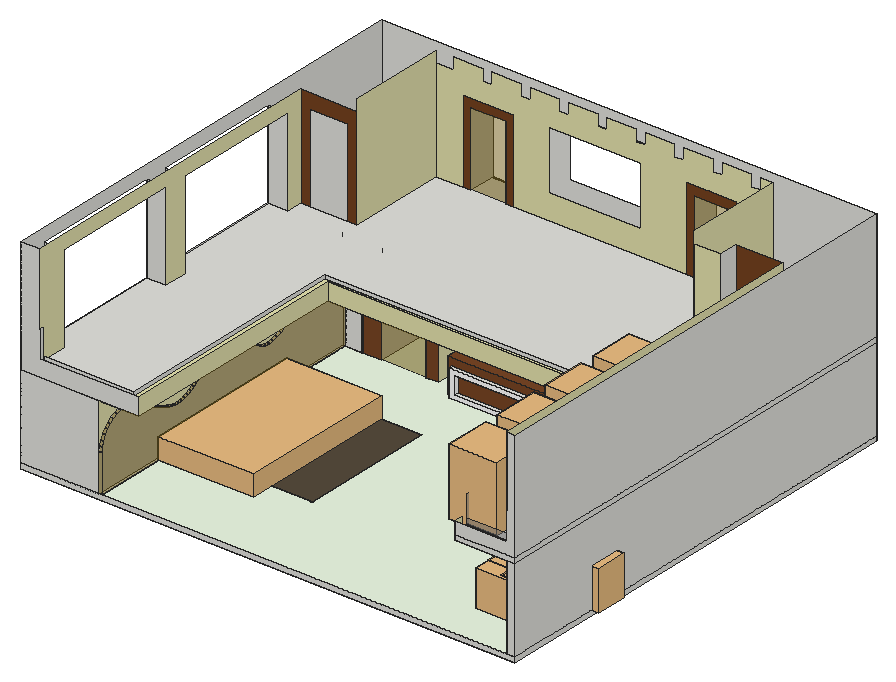
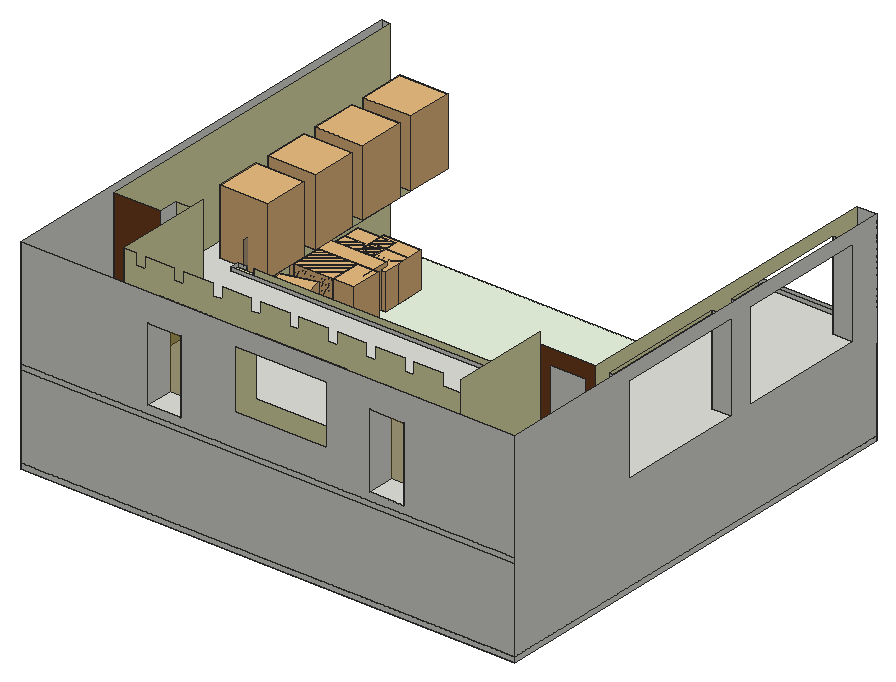
# SketchUp Ruby script. Lengths in inches.
U = 1.inch
M = Sketchup.active_model
def pt(a) = Geom::Point3d.new(a.map { |v| v * U })
def face(e, loops, mat)
  f = e.add_face(loops[0].map { |a| pt(a) })
  loops[1..].each { |l| e.add_face(l.map { |a| pt(a) }).erase! }
  f.material = f.back_material = mat if mat
  f
end
# faces: each face lists its corners as indices into pts; further lists are holes
def faces(e, pts, list, mat = nil) = list.each { |f| face(e, (f[0].is_a?(Array) ? f : [f]).map { |l| l.map { |i| pts[i] } }, mat) }
# xy, xz, yz: faces in a plane at the given z, y or x. An outline is a flat list of corners, or four numbers for a rectangle; further outlines are holes
def ring(l) = l.size == 4 ? [[l[0], l[1]], [l[2], l[1]], [l[2], l[3]], [l[0], l[3]]] : l.each_slice(2).to_a
def flat(e, list, mat, &to3) = list.each { |f| face(e, (f[0].is_a?(Array) ? f : [f]).map { |l| ring(l).map { |u, v| to3.(u, v) } }, mat) }
def xy(e, z, list, mat = nil) = flat(e, list, mat) { |x, y| [x, y, z] }
def xz(e, y, list, mat = nil) = flat(e, list, mat) { |x, z| [x, y, z] }
def yz(e, x, list, mat = nil) = flat(e, list, mat) { |y, z| [x, y, z] }
def lines(e, pts, list) = list.each { |a, b| e.add_line(pt(pts[a]), pt(pts[b])) }
# prism: a flat outline (further loops are holes) pulled along v
def prism(e, loops, v, mat = nil)
  f = face(e, loops, mat); d = Geom::Vector3d.new(v.map { |x| x * U })
  f.pushpull(f.normal.samedirection?(d) ? d.length : -d.length)
end
def box(e, o, s, mat = nil) = prism(e, [[o, [o[0] + s[0], o[1], o[2]], [o[0] + s[0], o[1] + s[1], o[2]], [o[0], o[1] + s[1], o[2]]]], [0, 0, s[2]], mat)
def at(x, y, z, deg = 0) = Geom::Transformation.translation(pt([x, y, z])) * Geom::Transformation.rotation(ORIGIN, Z_AXIS, deg.degrees)
def axes(o, x, y, z) = Geom::Transformation.new([*x, 0, *y, 0, *z, 0, *pt(o).to_a, 1])
def part(name) = M.definitions.add(name)
# library, detail: a bought-in or finely detailed component or shape, given as its bounding box
def library(name, o, s) = part(name).tap { |d| box(d.entities, o, s) }
def detail(e, o, s) = box(e.add_group.entities, o, s)
def put(e, d, t, mat = nil) = e.add_instance(d, t).tap { |i| i.material = mat if mat }
def group(e, t, mat = nil) = e.add_group.tap { |g| g.transformation = t; g.material = mat if mat }.entities
root = M.entities
M.materials.add("Generic").color = [229, 227, 174]
M.materials.add("[Carpet Diamond Olive]").color = [86, 76, 60]
M.materials.add("[Color M00]").color = [255, 255, 255]
M.materials.add("[Tile Limestone Large]").color = [236, 249, 228]
M.materials.add("[Translucent Glass Dark Green]").color = [135, 108, 20]
M.materials["[Translucent Glass Dark Green]"].alpha = 0.5
M.materials.add("[Translucent Glass Gray]").color = [128, 128, 128]
M.materials["[Translucent Glass Gray]"].alpha = 0.5
M.materials.add("[Wood Cherry Original]").color = [117, 66, 32]
M.materials.add("[Wood Veneer 01]").color = [120, 70, 37]
c1 = library("Group3\#1",[-238.15,54.18,0],[46.4,43.96,56.68])
c2 = library("Mesa PP75 Dining Table(beckup)",[0,0,0],[55.12,55.12,30.6875])
c3 = library("Plant+2 (1)",[-9.13,-9.52,0],[51.76,51.77,66.88])
c4 = library("Group\#6",[-0.47,-0.47,0],[175.35,198.73,37.5625])
c5 = library("1",[-11,-10.66,0],[22,21.32,33.52])
c6 = part("DDR842RVS01100X")
xy(c6.entities,0,[[-70.87,0,47.24,78.74]])
xy(c6.entities,0.39,[[-70.87,0,47.24,78.74]],"[Carpet Diamond Olive]")
xz(c6.entities,0,[[-70.87,0,47.24,0.39]])
xz(c6.entities,78.74,[[-70.87,0,47.24,0.39]])
yz(c6.entities,-70.87,[[0,0,78.74,0.39]])
yz(c6.entities,47.24,[[0,0,78.74,0.39]])
c7 = library("Flower_pot 07",[-1.21,-1.21,0],[8.32,8.32,4.71])
c8 = library("Plant",[-27.84,-31.84,-1.26],[68.28,70.82,154.38])
c9 = part("Group\#8")
xz(c9.entities,0,[[0,0,75.33,169.3125]],"[Translucent Glass Dark Green]")
xy(root,-12,[[0,0,1142.0625,1041.5]])
xy(root,0,[[0,0,182,0,182,701.375,227.9375,701.375,227.9375,701.68,228.24,701.68,228.24,701.375,273.88,701.375,273.88,831.5,375.13,831.5,375.13,701.375,404.03,701.375,404.03,830.0625,754.81,830.0625,754.81,849.8125,863.56,849.8125,863.56,701.375,931.8125,701.375,931.8125,828.25,1093.9375,828.25,1093.9375,701.375,1122.5625,701.375,1122.5625,0,1142.0625,0,1142.0625,1041.5,0,1041.5],[182,0,189.3125,701.375]])
xy(root,0,[[[189.3125,0,1122.5625,0,1122.5625,701.375,1093.9375,701.375,1093.9375,828.25,931.8125,828.25,931.8125,701.375,863.56,701.375,863.56,849.8125,754.81,849.8125,754.81,830.0625,404.03,830.0625,404.03,701.375,375.13,701.375,375.13,831.5,273.88,831.5,273.88,701.375,228.24,701.375,228.24,701.68,227.9375,701.68,227.9375,701.375,189.3125,701.375],[454.04,669.74,454.04,678.18,444.4,678.18,444.4,766.31,750.77,766.31,750.77,678.18,710.05,678.18,710.05,669.74]]],"[Tile Limestone Large]")
xy(root,11.125,[[467.72,669.74,710.05,678.18]])
xy(root,50.52,[[467.72,669.74,640.72,678.18]])
xy(root,61.64,[[454.04,669.74,640.72,678.18]])
xy(root,79.9375,[[444.4,678.18,750.77,766.31]],"[Wood Veneer 01]")
xy(root,133.0625,[[273.88,701.375,375.13,831.5]])
xy(root,141.1875,[[931.8125,701.375,1093.9375,828.25]])
xy(root,192,[[227.9375,701.375,228.24,701.68]])
xy(root,192,[[182,0,182,701.375,404.03,701.375,404.03,830.0625,754.81,830.0625,754.81,849.8125,863.56,849.8125,863.56,701.375,1122.5625,701.375,1122.5625,542.9375,274.125,542.9375,274.125,0],[1003,0,1122.5625,542.9375]],"Generic")
xy(root,222.75,[[45.5625,11.0625,253.5,11.0625,253.5,562.3125,1038.97,562.3125,1038.97,542.9375,1018.875,542.9375,1018.875,15.375,1122.5625,15.375,1122.5625,796.5,1014.875,796.5,1014.875,752.375,952.125,752.375,952.125,980.0625,847.11,980.0625,847.11,1041.5,771.78,1041.5,771.78,980.0625,335.28,980.0625,335.28,1041.5,255.99,1041.5,255.99,980.0625,175.5625,980.0625,175.5625,752.375,45.5625,752.375,45.5625,713.6,0,713.6,0,417.04,45.5625,417.04,45.5625,364.1,0,364.1,0,67.54,45.5625,67.54]])
xz(root,0,[[0,-12,1142.0625,0],[0,0,182,192],[1122.5625,0,1142.0625,192],[0,192,274.125,192,274.125,231.375,45.5625,231.375,45.5625,457.375,0,457.375],[1003,192,1142.0625,204],
  [1003,204,1142.0625,204,1142.0625,457.375,1122.5625,457.375,1122.5625,231.375,1003,231.375]])
xz(root,0,[[182,0,189.3125,86]],"[Translucent Glass Dark Green]")
xz(root,11.0625,[[45.5625,222.75,253.5,231.375]])
xz(root,15.375,[[1018.875,222.75,1122.5625,237.375]],"[Translucent Glass Gray]")
xz(root,67.54,[[0,222.75,45.5625,426.5625]])
xz(root,364.1,[[0,222.75,45.5625,426.5625]])
xz(root,417.04,[[0,222.75,45.5625,426.5625]])
xz(root,542.9375,[[1018.875,222.75,1038.97,231.375]])
xz(root,542.9375,[[274.125,192,1003,231.375]],"Generic")
xz(root,562.3125,[[253.5,222.75,1038.97,231.375]])
xz(root,669.74,[[454.04,0,710.05,0,710.05,11.125,467.72,11.125,467.72,50.52,640.72,50.52,640.72,61.64,454.04,61.64]],"[Color M00]")
xz(root,678.18,[[444.4,0,454.04,0,454.04,61.64,640.72,61.64,640.72,50.52,467.72,50.52,467.72,11.125,710.05,11.125,710.05,0,750.77,0,750.77,79.9375,444.4,79.9375]],"[Wood Veneer 01]")
xz(root,701.375,[[182,0,189.3125,132.8],[189.3125,0,227.9375,0,227.9375,192,182,192,182,132.8,189.3125,132.8]])
xz(root,701.375,[[863.56,0,911.78,192]],"Generic")
xz(root,701.375,[[911.78,0,931.8125,0,931.8125,141.1875,1093.9375,141.1875,1093.9375,0,1122.5625,0,1122.5625,192,911.78,192]],"[Wood Cherry Original]")
xz(root,701.375,[[228.24,0,273.88,0,273.88,133.0625,375.13,133.0625,375.13,0,404.03,0,404.03,192,228.24,192]],"[Wood Veneer 01]")
xz(root,701.68,[[227.9375,0,228.24,192]])
xz(root,713.6,[[0,222.75,45.5625,426.5625]])
xz(root,752.375,[[67.69,222.75,151.75,422.75]])
xz(root,752.375,[[952.125,222.75,1014.875,457.375]],"Generic")
xz(root,752.375,[[45.5625,222.75,67.69,222.75,67.69,422.75,151.75,422.75,151.75,222.75,175.5625,222.75,175.5625,457.375,45.5625,457.375]],"[Wood Cherry Original]")
xz(root,766.31,[[444.4,0,750.77,79.9375]])
xz(root,796.5,[[1014.875,222.75,1122.5625,457.375]],"[Wood Cherry Original]")
xz(root,828.25,[[931.8125,0,1093.9375,141.1875]])
xz(root,830.0625,[[404.03,39.25,754.81,45.5625],[404.03,78.375,754.81,84.6875],[404.03,117.5,754.81,123.8125],[404.03,156.625,754.81,162.9375],[404.03,162.9375,754.81,192]])
xz(root,830.0625,[[404.03,0,754.81,39.25],[404.03,45.5625,754.81,78.375],[404.03,84.6875,754.81,117.5],[404.03,123.8125,754.81,156.625]],"Generic")
xz(root,831.5,[[273.88,0,375.13,133.0625]])
xz(root,849.8125,[[754.81,0,863.56,39.29],[754.81,39.29,863.56,45.61],[754.81,78.4,863.56,84.72],[754.81,117.51,863.56,123.83],[754.81,156.625,863.56,162.9375]])
xz(root,849.8125,[[754.81,45.61,863.56,78.4],[754.81,84.72,863.56,117.51],[754.81,123.83,863.56,156.625],[754.81,162.9375,863.56,192]],"Generic")
xz(root,980.0625,[[[175.5625,222.75,236.76,222.75,236.76,413.27,354.51,413.27,354.51,222.75,750.57,222.75,750.57,413.27,868.32,413.27,868.32,222.75,952.125,222.75,952.125,483.5625,924.64,483.5625,924.64,457.375,902.01,457.375,902.01,483.5625,836.08,483.5625,836.08,457.375,813.45,457.375,813.45,483.5625,747.51,483.5625,747.51,457.375,724.89,457.375,724.89,483.5625,658.95,483.5625,658.95,457.375,636.33,457.375,636.33,483.5625,570.39,483.5625,570.39,457.375,547.76,457.375,547.76,483.5625,481.83,483.5625,481.83,457.375,459.2,457.375,459.2,483.5625,393.26,483.5625,393.26,457.375,370.64,457.375,370.64,483.5625,304.7,483.5625,304.7,457.375,282.08,457.375,282.08,483.5625,216.14,483.5625,216.14,457.375,175.5625,457.375],[434.63,279.55,646.76,416.17]]],"Generic")
xz(root,980.0625,[[236.76,222.75,255.99,222.75,255.99,394.04,335.28,394.04,335.28,222.75,354.51,222.75,354.51,413.27,236.76,413.27],[750.57,222.75,771.78,222.75,771.78,392.0625,847.11,392.0625,847.11,222.75,868.32,222.75,868.32,413.27,750.57,413.27]],"[Wood Cherry Original]")
xz(root,1041.5,[[0,-12,1142.0625,0],[0,0,1142.0625,192],[0,192,1142.0625,204],[[0,204,1142.0625,457.375],[434.63,279.55,646.76,416.17],[255.99,222.75,335.28,394.04],[771.78,222.75,847.11,392.0625]]])
yz(root,0,[[0,-12,1041.5,0],[[0,0,1041.5,457.375],[417.04,222.75,713.6,426.5625],[67.54,222.75,364.1,426.5625]]])
yz(root,45.5625,[[11.0625,222.75,67.54,222.75,67.54,426.5625,364.1,426.5625,364.1,222.75,417.04,222.75,417.04,426.5625,713.6,426.5625,713.6,222.75,752.375,222.75,752.375,457.375,0,457.375,0,293.625,11.0625,293.625]],"Generic")
yz(root,175.5625,[[752.375,222.75,980.0625,483.5625]],"Generic")
yz(root,182,[[0,0,0,86,1.01,97.52,4.02,108.68,8.92,119.14,15.58,128.59,23.79,136.73,33.28,143.32,43.79,148.14,54.97,151.0625,66.49,151.99,78,150.89,89.13,147.8,99.56,142.81,107.26,138.33,115.03,133.97,122.87,129.71,130.76,125.58,138.72,121.56,146.73,117.65,154.8,113.87,162.92,110.2,171.09,106.65,179.32,103.22,187.6,99.91,195.92,96.72,204.71,94.02,213.76,92.4,222.95,91.87,232.13,92.46,241.17,94.14,249.95,96.9,258.32,100.7,266.1875,105.47,273.42,111.16,279.91,117.68,285.57,124.92,290.32,132.8,298.0625,144.8,307.84,155.21,319.34,163.68,332.18,169.9375,345.93,173.78,360.16,175.07,374.38,173.78,388.13,169.9375,400.97,163.68,412.47,155.21,422.25,144.8,429.99,132.8,436.06,123.4,443.72,115.25,452.73,108.61,462.79,103.71,473.5625,100.7,484.71,99.6875,495.85,100.7,506.63,103.71,516.6875,108.61,525.69,115.25,533.36,123.4,539.42,132.8,548.4,146.72,559.74,158.78,573.07,168.61,587.96,175.86,603.91,180.3125,620.4,181.8125,636.89,180.3125,652.84,175.86,667.73,168.61,681.06,158.78,692.4,146.72,701.375,132.8,701.375,0]])
yz(root,182,[[0,86,1.01,97.52,4.02,108.68,8.92,119.14,15.58,128.59,23.79,136.73,33.28,143.32,43.79,148.14,54.97,151.0625,66.49,151.99,78,150.89,89.13,147.8,99.56,142.81,107.26,138.33,115.03,133.97,122.87,129.71,130.76,125.58,138.72,121.56,146.73,117.65,154.8,113.87,162.92,110.2,171.09,106.65,179.32,103.22,187.6,99.91,195.92,96.72,204.71,94.02,213.76,92.4,222.95,91.87,232.13,92.46,241.17,94.14,249.95,96.9,258.32,100.7,266.1875,105.47,273.42,111.16,279.91,117.68,285.57,124.92,290.32,132.8,298.0625,144.8,307.84,155.21,319.34,163.68,332.18,169.9375,345.93,173.78,360.16,175.07,374.38,173.78,388.13,169.9375,400.97,163.68,412.47,155.21,422.25,144.8,429.99,132.8,436.06,123.4,443.72,115.25,452.73,108.61,462.79,103.71,473.5625,100.7,484.71,99.6875,495.85,100.7,506.63,103.71,516.6875,108.61,525.69,115.25,533.36,123.4,539.42,132.8,548.4,146.72,559.74,158.78,573.07,168.61,587.96,175.86,603.91,180.3125,620.4,181.8125,636.89,180.3125,652.84,175.86,667.73,168.61,681.06,158.78,692.4,146.72,701.375,132.8,701.375,192,0,192]],"Generic")
yz(root,189.3125,[[0,0,701.375,0,701.375,132.8,692.4,146.72,681.06,158.78,667.73,168.61,652.84,175.86,636.89,180.3125,620.4,181.8125,603.91,180.3125,587.96,175.86,573.07,168.61,559.74,158.78,548.4,146.72,539.42,132.8,533.36,123.4,525.69,115.25,516.6875,108.61,506.63,103.71,495.85,100.7,484.71,99.6875,473.5625,100.7,462.79,103.71,452.73,108.61,443.72,115.25,436.06,123.4,429.99,132.8,422.25,144.8,412.47,155.21,400.97,163.68,388.13,169.9375,374.38,173.78,360.16,175.07,345.93,173.78,332.18,169.9375,319.34,163.68,307.84,155.21,298.0625,144.8,290.32,132.8,285.57,124.92,279.91,117.68,273.42,111.16,266.1875,105.47,258.32,100.7,249.95,96.9,241.17,94.14,232.13,92.46,222.95,91.87,213.76,92.4,204.71,94.02,195.92,96.72,187.6,99.91,179.32,103.22,171.09,106.65,162.92,110.2,154.8,113.87,146.73,117.65,138.72,121.56,130.76,125.58,122.87,129.71,115.03,133.97,107.26,138.33,99.56,142.81,89.13,147.8,78,150.89,66.49,151.99,54.97,151.0625,43.79,148.14,33.28,143.32,23.79,136.73,15.58,128.59,8.92,119.14,4.02,108.68,1.01,97.52,0,86]],"[Translucent Glass Dark Green]")
yz(root,227.9375,[[701.375,0,701.68,192]])
yz(root,228.24,[[701.375,0,701.68,192]])
yz(root,253.5,[[11.0625,222.75,562.3125,231.375]])
yz(root,255.99,[[980.0625,222.75,1041.5,394.04]])
yz(root,273.88,[[701.375,0,831.5,133.0625]])
yz(root,274.125,[[0,192,542.9375,231.375]],"Generic")
yz(root,335.28,[[980.0625,222.75,1041.5,394.04]])
yz(root,375.13,[[701.375,0,831.5,133.0625]])
yz(root,404.03,[[701.375,0,830.0625,192]],"Generic")
yz(root,444.4,[[678.18,0,766.31,79.9375]],"[Wood Veneer 01]")
yz(root,454.04,[[669.74,0,678.18,61.64]],"[Color M00]")
yz(root,467.72,[[669.74,11.125,678.18,50.52]],"[Color M00]")
yz(root,640.72,[[669.74,50.52,678.18,61.64]])
yz(root,710.05,[[669.74,0,678.18,11.125]])
yz(root,750.77,[[678.18,0,766.31,79.9375]],"[Wood Veneer 01]")
yz(root,754.81,[[830.0625,0,849.8125,123.8125],[830.0625,123.8125,849.8125,156.625],[830.0625,156.625,849.8125,162.9375],[830.0625,162.9375,849.8125,192]])
yz(root,771.78,[[980.0625,222.75,1041.5,392.0625]])
yz(root,847.11,[[980.0625,222.75,1041.5,392.0625]])
yz(root,863.56,[[701.375,0,849.8125,192]],"Generic")
yz(root,931.8125,[[701.375,0,828.25,141.1875]])
yz(root,952.125,[[752.375,222.75,980.0625,483.5625]],"Generic")
yz(root,1003,[[0,192,542.9375,231.375]],"Generic")
yz(root,1014.875,[[752.375,222.75,796.5,457.375]])
yz(root,1018.875,[[15.375,222.75,542.9375,222.75,542.9375,231.375,549.9375,231.375,549.9375,287.4375,15.375,287.4375]],"[Translucent Glass Gray]")
yz(root,1038.97,[[542.9375,222.75,562.3125,231.375]])
yz(root,1093.9375,[[701.375,0,828.25,141.1875]])
yz(root,1122.5625,[[0,0,701.375,192],[15.375,222.75,15.375,293.625,0,293.625,0,457.375,796.5,457.375,796.5,222.75]],"Generic")
yz(root,1142.0625,[[0,-12,1041.5,0],[0,0,1041.5,192],[0,192,1041.5,204],[0,204,1041.5,457.375]])
p = [[182,1.01,97.52],[182,0,86],[189.3125,0,86],[189.3125,1.01,97.52],[182,222.95,91.87],[182,213.76,92.4],
  [189.3125,213.76,92.4],[189.3125,222.95,91.87],[182,232.13,92.46],[189.3125,232.13,92.46],[182,204.71,94.02],[189.3125,204.71,94.02],
  [182,241.17,94.14],[189.3125,241.17,94.14],[182,195.92,96.72],[189.3125,195.92,96.72],[182,249.95,96.9],[189.3125,249.95,96.9],
  [182,187.6,99.91],[189.3125,187.6,99.91],[182,258.32,100.7],[189.3125,258.32,100.7],[182,4.02,108.68],[189.3125,4.02,108.68],
  [182,484.71,99.6875],[182,473.5625,100.7],[189.3125,473.5625,100.7],[189.3125,484.71,99.6875],[182,495.85,100.7],[189.3125,495.85,100.7],
  [182,179.32,103.22],[189.3125,179.32,103.22],[182,266.1875,105.47],[189.3125,266.1875,105.47],[182,462.79,103.71],[189.3125,462.79,103.71],
  [182,506.63,103.71],[189.3125,506.63,103.71],[182,171.09,106.65],[189.3125,171.09,106.65],[182,452.73,108.61],[189.3125,452.73,108.61],
  [182,516.6875,108.61],[189.3125,516.6875,108.61],[182,273.42,111.16],[189.3125,273.42,111.16],[182,162.92,110.2],[189.3125,162.92,110.2],
  [182,443.72,115.25],[189.3125,443.72,115.25],[182,525.69,115.25],[189.3125,525.69,115.25],[182,8.92,119.14],[189.3125,8.92,119.14],
  [182,154.8,113.87],[189.3125,154.8,113.87],[182,279.91,117.68],[189.3125,279.91,117.68],[182,146.73,117.65],[189.3125,146.73,117.65],
  [182,436.06,123.4],[189.3125,436.06,123.4],[182,533.36,123.4],[189.3125,533.36,123.4],[182,138.72,121.56],[189.3125,138.72,121.56],
  [182,285.57,124.92],[189.3125,285.57,124.92],[182,15.58,128.59],[189.3125,15.58,128.59],[182,130.76,125.58],[189.3125,130.76,125.58],
  [182,429.99,132.8],[189.3125,429.99,132.8],[182,539.42,132.8],[189.3125,539.42,132.8],[182,290.32,132.8],[189.3125,290.32,132.8],
  [182,122.87,129.71],[189.3125,122.87,129.71],[182,23.79,136.73],[189.3125,23.79,136.73],[182,115.03,133.97],[189.3125,115.03,133.97],
  [182,298.0625,144.8],[189.3125,298.0625,144.8],[182,422.25,144.8],[189.3125,422.25,144.8],[182,548.4,146.72],[189.3125,548.4,146.72],
  [182,701.375,132.8],[182,692.4,146.72],[189.3125,692.4,146.72],[189.3125,701.375,132.8],[182,107.26,138.33],[189.3125,107.26,138.33],
  [182,33.28,143.32],[189.3125,33.28,143.32],[182,99.56,142.81],[189.3125,99.56,142.81],[182,89.13,147.8],[189.3125,89.13,147.8],
  [182,43.79,148.14],[189.3125,43.79,148.14],[182,307.84,155.21],[189.3125,307.84,155.21],[182,412.47,155.21],[189.3125,412.47,155.21],
  [182,559.74,158.78],[189.3125,559.74,158.78],[182,681.06,158.78],[189.3125,681.06,158.78],[182,78,150.89],[189.3125,78,150.89],
  [182,54.97,151.0625],[189.3125,54.97,151.0625],[182,66.49,151.99],[189.3125,66.49,151.99],[182,319.34,163.68],[189.3125,319.34,163.68],
  [182,400.97,163.68],[189.3125,400.97,163.68],[182,573.07,168.61],[189.3125,573.07,168.61],[182,667.73,168.61],[189.3125,667.73,168.61],
  [182,332.18,169.9375],[189.3125,332.18,169.9375],[182,388.13,169.9375],[189.3125,388.13,169.9375],[182,587.96,175.86],[189.3125,587.96,175.86],
  [182,652.84,175.86],[189.3125,652.84,175.86],[182,345.93,173.78],[189.3125,345.93,173.78],[182,374.38,173.78],[189.3125,374.38,173.78],
  [182,360.16,175.07],[189.3125,360.16,175.07],[182,603.91,180.3125],[189.3125,603.91,180.3125],[182,636.89,180.3125],[189.3125,636.89,180.3125],
  [182,620.4,181.8125],[189.3125,620.4,181.8125],[182,701.375,192],[182,701.375,231.375],[274.125,701.375,192],[274.125,701.375,231.375]]
faces(root,p,[[0,1,2,3],[4,5,6,7],[8,4,7,9],[5,10,11,6],[12,8,9,13],[10,14,15,11],[16,12,13,17],[20,16,17,21],
  [22,0,3,23],[24,25,26,27],[28,24,27,29],[32,20,21,33],[25,34,35,26],[36,28,29,37],[34,40,41,35],[42,36,37,43],
  [44,32,33,45],[40,48,49,41],[50,42,43,51],[52,22,23,53],[56,44,45,57],[48,60,61,49],[62,50,51,63],[66,56,57,67],
  [68,52,53,69],[60,72,73,61],[74,62,63,75],[76,66,67,77],[80,68,69,81],[84,76,77,85],[72,86,87,73],[88,74,75,89],
  [90,91,92,93],[96,80,81,97],[98,100,101,99],[102,96,97,103],[104,84,85,105],[86,106,107,87],[108,88,89,109],[91,110,111,92],
  [100,112,113,101],[114,102,103,115],[112,116,117,113],[116,114,115,117],[118,104,105,119],[106,120,121,107],[122,108,109,123],[110,124,125,111],
  [126,118,119,127],[120,128,129,121],[130,122,123,131],[124,132,133,125],[134,126,127,135],[128,136,137,129],[138,134,135,139],[136,138,139,137],
  [140,130,131,141],[132,142,143,133],[144,140,141,145],[142,144,145,143]],"[Translucent Glass Dark Green]")
faces(root,p,[[14,18,19,15],[18,30,31,19],[30,38,39,31],[38,46,47,39],[46,54,55,47],[54,58,59,55],[58,64,65,59],[64,70,71,65],
  [70,78,79,71],[78,82,83,79],[82,94,95,83],[94,98,99,95]])
lines(root,p,[[146,147],[148,149]])
put(root,c1,axes([1696.49,89.61,-1.93],[2.98094,0,0],[0,1.63,0],[0,0,1.63]))
put(root,c2,at(313.48,335.47,0),"[Translucent Glass Gray]")
put(root,c3,axes([989.8,143.4375,0],[1.69136,0,0],[0,1.24,0],[0,0,1.24]))
put(root,c3,axes([989.8,106.4375,0],[1.69136,0,0],[0,1.24,0],[0,0,1.24]))
g1 = group(root,at(273.88,701.375,0))
xz(g1,0,[[0,0,101.25,133.0625]],"[Translucent Glass Dark Green]")
g2 = group(root,at(931.8125,701.375,0))
xz(g2,0,[[0,0,162.125,141.1875]],"[Translucent Glass Dark Green]")
put(root,c4,axes([187.3,164.79,0],[1.26,0,0],[0,1.8648,0],[0,0,1.26]))
put(root,c1,axes([1731.53,131.41,0],[2.98094,0,0],[0,1.63,0],[0,0,1.63]))
put(root,c3,axes([1042.92,151.82,0],[1.69136,0,0],[0,1.24,0],[0,0,1.24]))
put(root,c3,axes([1042.92,114.82,0],[1.69136,0,0],[0,1.24,0],[0,0,1.24]))
put(root,c1,axes([1683.28,131.41,0],[2.98094,0,0],[0,1.63,0],[0,0,1.63]))
put(root,c5,axes([1070.19,420.15,0],[0.68328,-2.55004,0],[3.51906,0.94293,0],[0,0,2.64]))
put(root,c5,axes([1070.19,347.28,0],[0.68328,-2.55004,0],[3.51906,0.94293,0],[0,0,2.64]))
put(root,c5,axes([1070.19,496.71,0],[0.68328,-2.55004,0],[3.51906,0.94293,0],[0,0,2.64]))
put(root,c6,axes([382.7,213.91,1.17],[2.541,0,0],[0,4.0053,0],[0,0,1]))
put(root,c7,axes([333.92,353.14,29.9375],[2.254,0,0],[0,2.254,0],[0,0,2.254]))
put(root,c8,axes([1019.15,66.84,219.42],[1.62,0,0],[0,1.485,0],[0,0,1]))
put(root,c8,axes([1019.15,204.59,219.42],[1.62,0,0],[0,1.485,0],[0,0,1]))
put(root,c8,axes([1019.15,342.34,219.42],[1.62,0,0],[0,1.485,0],[0,0,1]))
put(root,c8,axes([1019.15,480.09,219.42],[1.62,0,0],[0,1.485,0],[0,0,1]))
put(root,c9,at(771.78,980.0625,222.75))
put(root,c9,axes([255.99,980.0625,222.75],[1.05258,0,0],[0,1,0],[0,0,1.0117]))
